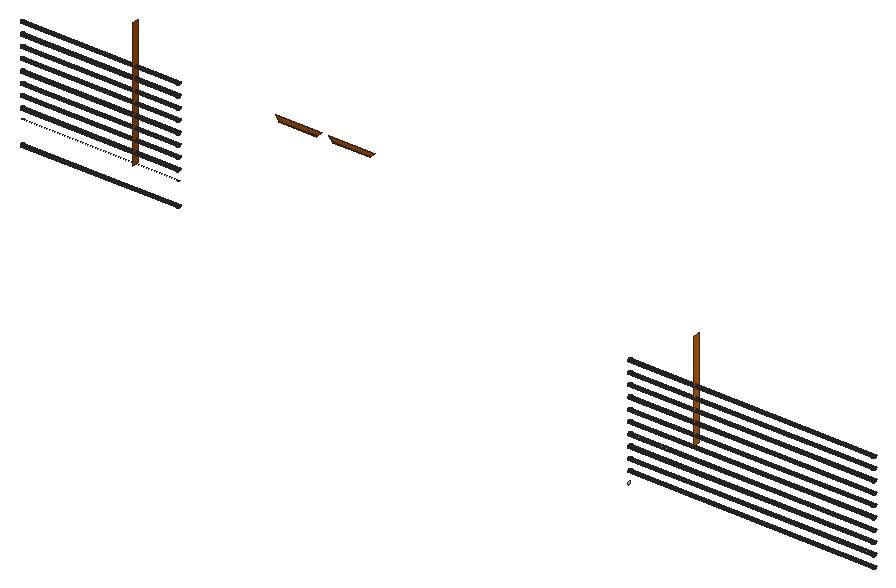
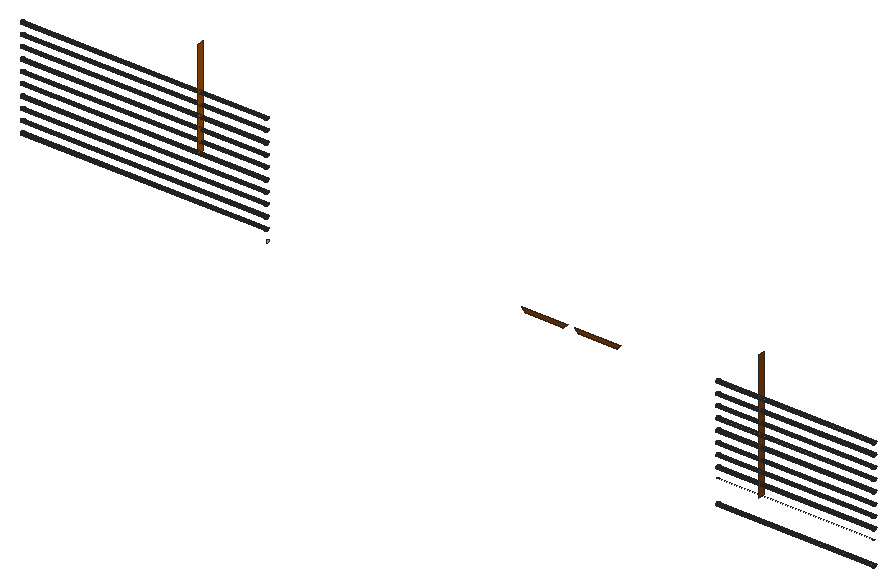
# SketchUp Ruby script. Lengths in inches.
U = 1.inch
M = Sketchup.active_model
def pt(a) = Geom::Point3d.new(a.map { |v| v * U })
def face(e, loops, mat)
  f = e.add_face(loops[0].map { |a| pt(a) })
  loops[1..].each { |l| e.add_face(l.map { |a| pt(a) }).erase! }
  f.material = f.back_material = mat if mat
  f
end
# faces: each face lists its corners as indices into pts; further lists are holes
def faces(e, pts, list, mat = nil) = list.each { |f| face(e, (f[0].is_a?(Array) ? f : [f]).map { |l| l.map { |i| pts[i] } }, mat) }
# xy, xz, yz: faces in a plane at the given z, y or x. An outline is a flat list of corners, or four numbers for a rectangle; further outlines are holes
def ring(l) = l.size == 4 ? [[l[0], l[1]], [l[2], l[1]], [l[2], l[3]], [l[0], l[3]]] : l.each_slice(2).to_a
def flat(e, list, mat, &to3) = list.each { |f| face(e, (f[0].is_a?(Array) ? f : [f]).map { |l| ring(l).map { |u, v| to3.(u, v) } }, mat) }
def xy(e, z, list, mat = nil) = flat(e, list, mat) { |x, y| [x, y, z] }
def xz(e, y, list, mat = nil) = flat(e, list, mat) { |x, z| [x, y, z] }
def yz(e, x, list, mat = nil) = flat(e, list, mat) { |y, z| [x, y, z] }
def lines(e, pts, list) = list.each { |a, b| e.add_line(pt(pts[a]), pt(pts[b])) }
# prism: a flat outline (further loops are holes) pulled along v
def prism(e, loops, v, mat = nil)
  f = face(e, loops, mat); d = Geom::Vector3d.new(v.map { |x| x * U })
  f.pushpull(f.normal.samedirection?(d) ? d.length : -d.length)
end
def box(e, o, s, mat = nil) = prism(e, [[o, [o[0] + s[0], o[1], o[2]], [o[0] + s[0], o[1] + s[1], o[2]], [o[0], o[1] + s[1], o[2]]]], [0, 0, s[2]], mat)
def at(x, y, z, deg = 0) = Geom::Transformation.translation(pt([x, y, z])) * Geom::Transformation.rotation(ORIGIN, Z_AXIS, deg.degrees)
def axes(o, x, y, z) = Geom::Transformation.new([*x, 0, *y, 0, *z, 0, *pt(o).to_a, 1])
def part(name) = M.definitions.add(name)
# library, detail: a bought-in or finely detailed component or shape, given as its bounding box
def library(name, o, s) = part(name).tap { |d| box(d.entities, o, s) }
def detail(e, o, s) = box(e.add_group.entities, o, s)
def put(e, d, t, mat = nil) = e.add_instance(d, t).tap { |i| i.material = mat if mat }
def group(e, t, mat = nil) = e.add_group.tap { |g| g.transformation = t; g.material = mat if mat }.entities
root = M.entities
M.materials.add("[0132_LightGray]").color = [169, 169, 169]
M.materials.add("[Wood Bamboo]").color = [195, 96, 5]
M.materials.add("[Wood Cherry Original]").color = [152, 68, 0]
xy(root,121.5,[[154,85.05,167.69,85.25],[173.29,85.05,186.99,85.25]])
xz(root,85.25,[[154,121.5,167.69,121.5,169.19,123,152.5,123],[173.29,121.5,186.99,121.5,188.49,123,171.79,123]],"[Wood Cherry Original]")
yz(root,103.25,[[82.25,90.51,84.25,137.01]],"[Wood Cherry Original]")
yz(root,316.01,[[41.28,79.71,41.15,79.73,41.03,79.78,40.93,79.86,40.85,79.96,40.8,80.08,40.78,80.21,40.8,80.34,40.85,80.46,40.93,80.57,41.03,80.65,41.15,80.7,41.28,80.71,41.41,80.7,41.53,80.65,41.63,80.57,41.71,80.46,41.76,80.34,41.78,80.21,41.76,80.08,41.71,79.96,41.63,79.86,41.53,79.78,41.41,79.73]])
yz(root,340.01,[[40.5625,100.9,43,136.59]],"[Wood Bamboo]")
p = [[119.25,83,82.03],[119.25,82.9,82.11],[61.9375,82.9,82.11],[61.9375,83,82.03],[119.25,83.12,81.98],[61.9375,83.12,81.98],
  [119.25,83.25,81.96],[61.9375,83.25,81.96],[119.25,83.38,81.98],[61.9375,83.38,81.98],[119.25,83.5,82.03],[61.9375,83.5,82.03],
  [119.25,83.6,82.11],[61.9375,83.6,82.11],[119.25,82.82,82.21],[61.9375,82.82,82.21],[119.25,83.68,82.21],[61.9375,83.68,82.21],
  [119.25,82.77,82.34],[61.9375,82.77,82.34],[119.25,83.73,82.34],[61.9375,83.73,82.34],[119.25,82.75,82.46],[61.9375,82.75,82.46],
  [119.25,83.75,82.46],[61.9375,83.75,82.46],[119.25,82.77,82.59],[61.9375,82.77,82.59],[119.25,83.73,82.59],[61.9375,83.73,82.59],
  [119.25,82.82,82.71],[61.9375,82.82,82.71],[119.25,83.68,82.71],[61.9375,83.68,82.71],[119.25,82.9,82.82],[61.9375,82.9,82.82],
  [119.25,83.6,82.82],[61.9375,83.6,82.82],[119.25,83,82.9],[61.9375,83,82.9],[119.25,83.5,82.9],[61.9375,83.5,82.9],
  [119.25,83.12,82.95],[61.9375,83.12,82.95],[119.25,83.25,82.96],[61.9375,83.25,82.96],[119.25,83.38,82.95],[61.9375,83.38,82.95],
  [316.01,41.03,83.78],[316.01,41.15,83.73],[405.26,41.15,83.73],[405.26,41.03,83.78],[316.01,41.28,83.71],[405.26,41.28,83.71],
  [316.01,41.41,83.73],[405.26,41.41,83.73],[316.01,41.53,83.78],[405.26,41.53,83.78],[316.01,40.93,83.86],[405.26,40.93,83.86],
  [316.01,41.63,83.86],[405.26,41.63,83.86],[316.01,40.85,83.96],[405.26,40.85,83.96],[316.01,41.71,83.96],[405.26,41.71,83.96],
  [316.01,40.8,84.08],[405.26,40.8,84.08],[316.01,41.76,84.08],[405.26,41.76,84.08],[316.01,40.78,84.21],[405.26,40.78,84.21],
  [316.01,41.78,84.21],[405.26,41.78,84.21],[316.01,40.8,84.34],[405.26,40.8,84.34],[316.01,41.76,84.34],[405.26,41.76,84.34],
  [316.01,40.85,84.46],[405.26,40.85,84.46],[316.01,41.71,84.46],[405.26,41.71,84.46],[316.01,40.93,84.57],[405.26,40.93,84.57],
  [316.01,41.63,84.57],[405.26,41.63,84.57],[316.01,41.03,84.65],[405.26,41.03,84.65],[316.01,41.15,84.7],[405.26,41.15,84.7],
  [316.01,41.53,84.65],[316.01,41.41,84.7],[405.26,41.41,84.7],[405.26,41.53,84.65],[316.01,41.28,84.71],[405.26,41.28,84.71],
  [316.01,41.03,87.78],[316.01,41.15,87.73],[405.26,41.15,87.73],[405.26,41.03,87.78],[316.01,41.28,87.71],[405.26,41.28,87.71],
  [316.01,41.41,87.73],[405.26,41.41,87.73],[316.01,41.53,87.78],[405.26,41.53,87.78],[316.01,40.93,87.86],[405.26,40.93,87.86],
  [316.01,41.63,87.86],[405.26,41.63,87.86],[316.01,40.85,87.96],[405.26,40.85,87.96],[316.01,41.71,87.96],[405.26,41.71,87.96],
  [316.01,40.8,88.08],[405.26,40.8,88.08],[316.01,41.76,88.08],[405.26,41.76,88.08],[316.01,40.78,88.21],[405.26,40.78,88.21],
  [316.01,41.78,88.21],[405.26,41.78,88.21],[316.01,40.8,88.34],[405.26,40.8,88.34],[316.01,41.76,88.34],[405.26,41.76,88.34],
  [316.01,40.85,88.46],[405.26,40.85,88.46],[316.01,41.71,88.46],[405.26,41.71,88.46],[316.01,40.93,88.57],[405.26,40.93,88.57],
  [316.01,41.63,88.57],[405.26,41.63,88.57],[316.01,41.03,88.65],[405.26,41.03,88.65],[316.01,41.15,88.7],[405.26,41.15,88.7],
  [316.01,41.53,88.65],[316.01,41.41,88.7],[405.26,41.41,88.7],[405.26,41.53,88.65],[316.01,41.28,88.71],[405.26,41.28,88.71],
  [119.25,83.25,90.96],[119.25,83.38,90.95],[61.9375,83.38,90.95],[61.9375,83.25,90.96],[316.01,41.03,91.78],[316.01,41.15,91.73],
  [405.26,41.15,91.73],[405.26,41.03,91.78],[316.01,41.28,91.71],[405.26,41.28,91.71],[316.01,41.41,91.73],[405.26,41.41,91.73],
  [316.01,41.53,91.78],[405.26,41.53,91.78],[316.01,40.93,91.86],[405.26,40.93,91.86],[316.01,41.63,91.86],[405.26,41.63,91.86],
  [316.01,40.85,91.96],[405.26,40.85,91.96],[316.01,41.71,91.96],[405.26,41.71,91.96],[316.01,40.8,92.08],[405.26,40.8,92.08],
  [316.01,41.76,92.08],[405.26,41.76,92.08],[316.01,40.78,92.21],[405.26,40.78,92.21],[316.01,41.78,92.21],[405.26,41.78,92.21],
  [316.01,40.8,92.34],[405.26,40.8,92.34],[316.01,41.76,92.34],[405.26,41.76,92.34],[316.01,40.85,92.46],[405.26,40.85,92.46],
  [316.01,41.71,92.46],[405.26,41.71,92.46],[316.01,40.93,92.57],[405.26,40.93,92.57],[316.01,41.63,92.57],[405.26,41.63,92.57],
  [316.01,41.03,92.65],[405.26,41.03,92.65],[316.01,41.15,92.7],[405.26,41.15,92.7],[316.01,41.53,92.65],[316.01,41.41,92.7],
  [405.26,41.41,92.7],[405.26,41.53,92.65],[316.01,41.28,92.71],[405.26,41.28,92.71],[119.25,83,94.03],[119.25,82.9,94.11],
  [61.9375,82.9,94.11],[61.9375,83,94.03],[119.25,83.12,93.98],[61.9375,83.12,93.98],[119.25,83.25,93.96],[61.9375,83.25,93.96],
  [119.25,83.38,93.98],[61.9375,83.38,93.98],[119.25,83.5,94.03],[61.9375,83.5,94.03],[119.25,83.6,94.11],[61.9375,83.6,94.11],
  [119.25,82.82,94.21],[61.9375,82.82,94.21],[119.25,83.68,94.21],[61.9375,83.68,94.21],[119.25,82.77,94.34],[61.9375,82.77,94.34],
  [119.25,83.73,94.34],[61.9375,83.73,94.34],[119.25,82.75,94.46],[61.9375,82.75,94.46],[119.25,83.75,94.46],[61.9375,83.75,94.46],
  [119.25,82.77,94.59],[61.9375,82.77,94.59],[119.25,83.73,94.59],[61.9375,83.73,94.59],[119.25,82.82,94.71],[61.9375,82.82,94.71],
  [119.25,83.68,94.71],[61.9375,83.68,94.71],[119.25,82.9,94.82],[61.9375,82.9,94.82],[119.25,83.6,94.82],[61.9375,83.6,94.82],
  [119.25,83,94.9],[61.9375,83,94.9],[119.25,83.5,94.9],[61.9375,83.5,94.9],[119.25,83.12,94.95],[61.9375,83.12,94.95],
  [119.25,83.25,94.96],[61.9375,83.25,94.96],[119.25,83.38,94.95],[61.9375,83.38,94.95],[316.01,41.03,95.78],[316.01,41.15,95.73],
  [405.26,41.15,95.73],[405.26,41.03,95.78],[316.01,41.28,95.71],[405.26,41.28,95.71],[316.01,41.41,95.73],[405.26,41.41,95.73],
  [316.01,41.53,95.78],[405.26,41.53,95.78],[316.01,40.93,95.86],[405.26,40.93,95.86],[316.01,41.63,95.86],[405.26,41.63,95.86],
  [316.01,40.85,95.96],[405.26,40.85,95.96],[316.01,41.71,95.96],[405.26,41.71,95.96],[316.01,40.8,96.08],[405.26,40.8,96.08],
  [316.01,41.76,96.08],[405.26,41.76,96.08],[316.01,40.78,96.21],[405.26,40.78,96.21],[316.01,41.78,96.21],[405.26,41.78,96.21],
  [316.01,40.8,96.34],[405.26,40.8,96.34],[316.01,41.76,96.34],[405.26,41.76,96.34],[316.01,40.85,96.46],[405.26,40.85,96.46],
  [316.01,41.71,96.46],[405.26,41.71,96.46],[316.01,40.93,96.57],[405.26,40.93,96.57],[316.01,41.63,96.57],[405.26,41.63,96.57],
  [316.01,41.03,96.65],[405.26,41.03,96.65],[316.01,41.15,96.7],[405.26,41.15,96.7],[316.01,41.53,96.65],[316.01,41.41,96.7],
  [405.26,41.41,96.7],[405.26,41.53,96.65],[316.01,41.28,96.71],[405.26,41.28,96.71],[119.25,83,98.03],[119.25,82.9,98.11],
  [61.9375,82.9,98.11],[61.9375,83,98.03],[119.25,83.12,97.98],[61.9375,83.12,97.98],[119.25,83.25,97.96],[61.9375,83.25,97.96],
  [119.25,83.38,97.98],[61.9375,83.38,97.98],[119.25,83.5,98.03],[61.9375,83.5,98.03],[119.25,83.6,98.11],[61.9375,83.6,98.11],
  [119.25,82.82,98.21],[61.9375,82.82,98.21],[119.25,83.68,98.21],[61.9375,83.68,98.21],[119.25,82.77,98.34],[61.9375,82.77,98.34],
  [119.25,83.73,98.34],[61.9375,83.73,98.34],[119.25,82.75,98.46],[61.9375,82.75,98.46],[119.25,83.75,98.46],[61.9375,83.75,98.46],
  [119.25,82.77,98.59],[61.9375,82.77,98.59],[119.25,83.73,98.59],[61.9375,83.73,98.59],[119.25,82.82,98.71],[61.9375,82.82,98.71],
  [119.25,83.68,98.71],[61.9375,83.68,98.71],[119.25,82.9,98.82],[61.9375,82.9,98.82],[119.25,83.6,98.82],[61.9375,83.6,98.82],
  [119.25,83,98.9],[61.9375,83,98.9],[119.25,83.5,98.9],[61.9375,83.5,98.9],[119.25,83.12,98.95],[61.9375,83.12,98.95],
  [119.25,83.25,98.96],[61.9375,83.25,98.96],[119.25,83.38,98.95],[61.9375,83.38,98.95],[316.01,41.03,99.78],[316.01,41.15,99.73],
  [405.26,41.15,99.73],[405.26,41.03,99.78],[316.01,41.28,99.71],[405.26,41.28,99.71],[316.01,41.41,99.73],[405.26,41.41,99.73],
  [316.01,41.53,99.78],[405.26,41.53,99.78],[316.01,40.93,99.86],[405.26,40.93,99.86],[316.01,41.63,99.86],[405.26,41.63,99.86],
  [316.01,40.85,99.96],[405.26,40.85,99.96],[316.01,41.71,99.96],[405.26,41.71,99.96],[316.01,40.8,100.08],[405.26,40.8,100.08],
  [316.01,41.76,100.08],[405.26,41.76,100.08],[316.01,40.78,100.21],[405.26,40.78,100.21],[316.01,41.78,100.21],[405.26,41.78,100.21],
  [316.01,40.8,100.34],[405.26,40.8,100.34],[316.01,41.76,100.34],[405.26,41.76,100.34],[316.01,40.85,100.46],[405.26,40.85,100.46],
  [316.01,41.71,100.46],[405.26,41.71,100.46],[316.01,40.93,100.57],[405.26,40.93,100.57],[316.01,41.63,100.57],[405.26,41.63,100.57],
  [316.01,41.03,100.65],[405.26,41.03,100.65],[316.01,41.15,100.7],[405.26,41.15,100.7],[316.01,41.53,100.65],[316.01,41.41,100.7],
  [405.26,41.41,100.7],[405.26,41.53,100.65],[316.01,41.28,100.71],[405.26,41.28,100.71],[119.25,83,102.03],[119.25,82.9,102.11],
  [61.9375,82.9,102.11],[61.9375,83,102.03],[119.25,83.12,101.98],[61.9375,83.12,101.98],[119.25,83.25,101.96],[61.9375,83.25,101.96],
  [119.25,83.38,101.98],[61.9375,83.38,101.98],[119.25,83.5,102.03],[61.9375,83.5,102.03],[119.25,83.6,102.11],[61.9375,83.6,102.11],
  [119.25,82.82,102.21],[61.9375,82.82,102.21],[119.25,83.68,102.21],[61.9375,83.68,102.21],[119.25,82.77,102.34],[61.9375,82.77,102.34],
  [119.25,83.73,102.34],[61.9375,83.73,102.34],[119.25,82.75,102.46],[61.9375,82.75,102.46],[119.25,83.75,102.46],[61.9375,83.75,102.46],
  [119.25,82.77,102.59],[61.9375,82.77,102.59],[119.25,83.73,102.59],[61.9375,83.73,102.59],[119.25,82.82,102.71],[61.9375,82.82,102.71],
  [119.25,83.68,102.71],[61.9375,83.68,102.71],[119.25,82.9,102.82],[61.9375,82.9,102.82],[119.25,83.6,102.82],[61.9375,83.6,102.82],
  [119.25,83,102.9],[61.9375,83,102.9],[119.25,83.5,102.9],[61.9375,83.5,102.9],[119.25,83.12,102.95],[61.9375,83.12,102.95],
  [119.25,83.25,102.96],[61.9375,83.25,102.96],[119.25,83.38,102.95],[61.9375,83.38,102.95],[316.01,41.03,103.78],[316.01,41.15,103.73],
  [405.26,41.15,103.73],[405.26,41.03,103.78],[316.01,41.28,103.71],[405.26,41.28,103.71],[316.01,41.41,103.73],[405.26,41.41,103.73],
  [316.01,41.53,103.78],[405.26,41.53,103.78],[316.01,40.93,103.86],[405.26,40.93,103.86],[316.01,41.63,103.86],[405.26,41.63,103.86],
  [316.01,40.85,103.96],[405.26,40.85,103.96],[316.01,41.71,103.96],[405.26,41.71,103.96],[316.01,40.8,104.08],[405.26,40.8,104.08],
  [316.01,41.76,104.08],[405.26,41.76,104.08],[316.01,40.78,104.21],[405.26,40.78,104.21],[316.01,41.78,104.21],[405.26,41.78,104.21],
  [316.01,40.8,104.34],[405.26,40.8,104.34],[316.01,41.76,104.34],[405.26,41.76,104.34],[316.01,40.85,104.46],[405.26,40.85,104.46],
  [316.01,41.71,104.46],[405.26,41.71,104.46],[316.01,40.93,104.57],[405.26,40.93,104.57],[316.01,41.63,104.57],[405.26,41.63,104.57],
  [316.01,41.03,104.65],[405.26,41.03,104.65],[316.01,41.15,104.7],[405.26,41.15,104.7],[316.01,41.53,104.65],[316.01,41.41,104.7],
  [405.26,41.41,104.7],[405.26,41.53,104.65],[316.01,41.28,104.71],[405.26,41.28,104.71],[119.25,83,106.03],[119.25,82.9,106.11],
  [61.9375,82.9,106.11],[61.9375,83,106.03],[119.25,83.12,105.98],[61.9375,83.12,105.98],[119.25,83.25,105.96],[61.9375,83.25,105.96],
  [119.25,83.38,105.98],[61.9375,83.38,105.98],[119.25,83.5,106.03],[61.9375,83.5,106.03],[119.25,83.6,106.11],[61.9375,83.6,106.11],
  [119.25,82.82,106.21],[61.9375,82.82,106.21],[119.25,83.68,106.21],[61.9375,83.68,106.21],[119.25,82.77,106.34],[61.9375,82.77,106.34],
  [119.25,83.73,106.34],[61.9375,83.73,106.34],[119.25,82.75,106.46],[61.9375,82.75,106.46],[119.25,83.75,106.46],[61.9375,83.75,106.46],
  [119.25,82.77,106.59],[61.9375,82.77,106.59],[119.25,83.73,106.59],[61.9375,83.73,106.59],[119.25,82.82,106.71],[61.9375,82.82,106.71],
  [119.25,83.68,106.71],[61.9375,83.68,106.71],[119.25,82.9,106.82],[61.9375,82.9,106.82],[119.25,83.6,106.82],[61.9375,83.6,106.82],
  [119.25,83,106.9],[61.9375,83,106.9],[119.25,83.5,106.9],[61.9375,83.5,106.9],[119.25,83.12,106.95],[61.9375,83.12,106.95],
  [119.25,83.25,106.96],[61.9375,83.25,106.96],[119.25,83.38,106.95],[61.9375,83.38,106.95],[316.01,41.03,107.78],[316.01,41.15,107.73],
  [405.26,41.15,107.73],[405.26,41.03,107.78],[316.01,41.28,107.71],[405.26,41.28,107.71],[316.01,41.41,107.73],[405.26,41.41,107.73],
  [316.01,41.53,107.78],[405.26,41.53,107.78],[316.01,40.93,107.86],[405.26,40.93,107.86],[316.01,41.63,107.86],[405.26,41.63,107.86],
  [316.01,40.85,107.96],[405.26,40.85,107.96],[316.01,41.71,107.96],[405.26,41.71,107.96],[316.01,40.8,108.08],[405.26,40.8,108.08],
  [316.01,41.76,108.08],[405.26,41.76,108.08],[316.01,40.78,108.21],[405.26,40.78,108.21],[316.01,41.78,108.21],[405.26,41.78,108.21],
  [316.01,40.8,108.34],[405.26,40.8,108.34],[316.01,41.76,108.34],[405.26,41.76,108.34],[316.01,40.85,108.46],[405.26,40.85,108.46],
  [316.01,41.71,108.46],[405.26,41.71,108.46],[316.01,40.93,108.57],[405.26,40.93,108.57],[316.01,41.63,108.57],[405.26,41.63,108.57],
  [316.01,41.03,108.65],[405.26,41.03,108.65],[316.01,41.15,108.7],[405.26,41.15,108.7],[316.01,41.53,108.65],[316.01,41.41,108.7],
  [405.26,41.41,108.7],[405.26,41.53,108.65],[316.01,41.28,108.71],[405.26,41.28,108.71],[119.25,83,110.03],[119.25,82.9,110.11],
  [61.9375,82.9,110.11],[61.9375,83,110.03],[119.25,83.12,109.98],[61.9375,83.12,109.98],[119.25,83.25,109.96],[61.9375,83.25,109.96],
  [119.25,83.38,109.98],[61.9375,83.38,109.98],[119.25,83.5,110.03],[61.9375,83.5,110.03],[119.25,83.6,110.11],[61.9375,83.6,110.11],
  [119.25,82.82,110.21],[61.9375,82.82,110.21],[119.25,83.68,110.21],[61.9375,83.68,110.21],[119.25,82.77,110.34],[61.9375,82.77,110.34],
  [119.25,83.73,110.34],[61.9375,83.73,110.34],[119.25,82.75,110.46],[61.9375,82.75,110.46],[119.25,83.75,110.46],[61.9375,83.75,110.46],
  [119.25,82.77,110.59],[61.9375,82.77,110.59],[119.25,83.73,110.59],[61.9375,83.73,110.59],[119.25,82.82,110.71],[61.9375,82.82,110.71],
  [119.25,83.68,110.71],[61.9375,83.68,110.71],[119.25,82.9,110.82],[61.9375,82.9,110.82],[119.25,83.6,110.82],[61.9375,83.6,110.82],
  [119.25,83,110.9],[61.9375,83,110.9],[119.25,83.5,110.9],[61.9375,83.5,110.9],[119.25,83.12,110.95],[61.9375,83.12,110.95],
  [119.25,83.25,110.96],[61.9375,83.25,110.96],[119.25,83.38,110.95],[61.9375,83.38,110.95],[316.01,41.03,111.78],[316.01,41.15,111.73],
  [405.26,41.15,111.73],[405.26,41.03,111.78],[316.01,41.28,111.71],[405.26,41.28,111.71],[316.01,41.41,111.73],[405.26,41.41,111.73],
  [316.01,41.53,111.78],[405.26,41.53,111.78],[316.01,40.93,111.86],[405.26,40.93,111.86],[316.01,41.63,111.86],[405.26,41.63,111.86],
  [316.01,40.85,111.96],[405.26,40.85,111.96],[316.01,41.71,111.96],[405.26,41.71,111.96],[316.01,40.8,112.08],[405.26,40.8,112.08],
  [316.01,41.76,112.08],[405.26,41.76,112.08],[316.01,40.78,112.21],[405.26,40.78,112.21],[316.01,41.78,112.21],[405.26,41.78,112.21],
  [316.01,40.8,112.34],[405.26,40.8,112.34],[316.01,41.76,112.34],[405.26,41.76,112.34],[316.01,40.85,112.46],[405.26,40.85,112.46],
  [316.01,41.71,112.46],[405.26,41.71,112.46],[316.01,40.93,112.57],[405.26,40.93,112.57],[316.01,41.63,112.57],[405.26,41.63,112.57],
  [316.01,41.03,112.65],[405.26,41.03,112.65],[316.01,41.15,112.7],[405.26,41.15,112.7],[316.01,41.53,112.65],[316.01,41.41,112.7],
  [405.26,41.41,112.7],[405.26,41.53,112.65],[316.01,41.28,112.71],[405.26,41.28,112.71],[119.25,83,114.03],[119.25,82.9,114.11],
  [61.9375,82.9,114.11],[61.9375,83,114.03],[119.25,83.12,113.98],[61.9375,83.12,113.98],[119.25,83.25,113.96],[61.9375,83.25,113.96],
  [119.25,83.38,113.98],[61.9375,83.38,113.98],[119.25,83.5,114.03],[61.9375,83.5,114.03],[119.25,83.6,114.11],[61.9375,83.6,114.11],
  [119.25,82.82,114.21],[61.9375,82.82,114.21],[119.25,83.68,114.21],[61.9375,83.68,114.21],[119.25,82.77,114.34],[61.9375,82.77,114.34],
  [119.25,83.73,114.34],[61.9375,83.73,114.34],[119.25,82.75,114.46],[61.9375,82.75,114.46],[119.25,83.75,114.46],[61.9375,83.75,114.46],
  [119.25,82.77,114.59],[61.9375,82.77,114.59],[119.25,83.73,114.59],[61.9375,83.73,114.59],[119.25,82.82,114.71],[61.9375,82.82,114.71],
  [119.25,83.68,114.71],[61.9375,83.68,114.71],[119.25,82.9,114.82],[61.9375,82.9,114.82],[119.25,83.6,114.82],[61.9375,83.6,114.82],
  [119.25,83,114.9],[61.9375,83,114.9],[119.25,83.5,114.9],[61.9375,83.5,114.9],[119.25,83.12,114.95],[61.9375,83.12,114.95],
  [119.25,83.25,114.96],[61.9375,83.25,114.96],[119.25,83.38,114.95],[61.9375,83.38,114.95],[316.01,41.03,115.78],[316.01,41.15,115.73],
  [405.26,41.15,115.73],[405.26,41.03,115.78],[316.01,41.28,115.71],[405.26,41.28,115.71],[316.01,41.41,115.73],[405.26,41.41,115.73],
  [316.01,41.53,115.78],[405.26,41.53,115.78],[316.01,40.93,115.86],[405.26,40.93,115.86],[316.01,41.63,115.86],[405.26,41.63,115.86],
  [316.01,40.85,115.96],[405.26,40.85,115.96],[316.01,41.71,115.96],[405.26,41.71,115.96],[316.01,40.8,116.08],[405.26,40.8,116.08],
  [316.01,41.76,116.08],[405.26,41.76,116.08],[316.01,40.78,116.21],[405.26,40.78,116.21],[316.01,41.78,116.21],[405.26,41.78,116.21],
  [316.01,40.8,116.34],[405.26,40.8,116.34],[316.01,41.76,116.34],[405.26,41.76,116.34],[316.01,40.85,116.46],[405.26,40.85,116.46],
  [316.01,41.71,116.46],[405.26,41.71,116.46],[316.01,40.93,116.57],[405.26,40.93,116.57],[316.01,41.63,116.57],[405.26,41.63,116.57],
  [316.01,41.03,116.65],[405.26,41.03,116.65],[316.01,41.15,116.7],[405.26,41.15,116.7],[316.01,41.53,116.65],[316.01,41.41,116.7],
  [405.26,41.41,116.7],[405.26,41.53,116.65],[316.01,41.28,116.71],[405.26,41.28,116.71],[119.25,83,118.03],[119.25,82.9,118.11],
  [61.9375,82.9,118.11],[61.9375,83,118.03],[119.25,83.12,117.98],[61.9375,83.12,117.98],[119.25,83.25,117.96],[61.9375,83.25,117.96],
  [119.25,83.38,117.98],[61.9375,83.38,117.98],[119.25,83.5,118.03],[61.9375,83.5,118.03],[119.25,83.6,118.11],[61.9375,83.6,118.11],
  [119.25,82.82,118.21],[61.9375,82.82,118.21],[119.25,83.68,118.21],[61.9375,83.68,118.21],[119.25,82.77,118.34],[61.9375,82.77,118.34],
  [119.25,83.73,118.34],[61.9375,83.73,118.34],[119.25,82.75,118.46],[61.9375,82.75,118.46],[119.25,83.75,118.46],[61.9375,83.75,118.46],
  [119.25,82.77,118.59],[61.9375,82.77,118.59],[119.25,83.73,118.59],[61.9375,83.73,118.59],[119.25,82.82,118.71],[61.9375,82.82,118.71],
  [119.25,83.68,118.71],[61.9375,83.68,118.71],[119.25,82.9,118.82],[61.9375,82.9,118.82],[119.25,83.6,118.82],[61.9375,83.6,118.82],
  [119.25,83,118.9],[61.9375,83,118.9],[119.25,83.5,118.9],[61.9375,83.5,118.9],[119.25,83.12,118.95],[61.9375,83.12,118.95],
  [119.25,83.25,118.96],[61.9375,83.25,118.96],[119.25,83.38,118.95],[61.9375,83.38,118.95],[316.01,41.03,119.78],[316.01,41.15,119.73],
  [405.26,41.15,119.73],[405.26,41.03,119.78],[316.01,41.28,119.71],[405.26,41.28,119.71],[316.01,41.41,119.73],[405.26,41.41,119.73],
  [316.01,41.53,119.78],[405.26,41.53,119.78],[316.01,40.93,119.86],[405.26,40.93,119.86],[316.01,41.63,119.86],[405.26,41.63,119.86],
  [316.01,40.85,119.96],[405.26,40.85,119.96],[316.01,41.71,119.96],[405.26,41.71,119.96],[316.01,40.8,120.08],[405.26,40.8,120.08],
  [316.01,41.76,120.08],[405.26,41.76,120.08],[316.01,40.78,120.21],[405.26,40.78,120.21],[316.01,41.78,120.21],[405.26,41.78,120.21],
  [316.01,40.8,120.34],[405.26,40.8,120.34],[316.01,41.76,120.34],[405.26,41.76,120.34],[316.01,40.85,120.46],[405.26,40.85,120.46],
  [316.01,41.71,120.46],[405.26,41.71,120.46],[316.01,40.93,120.57],[405.26,40.93,120.57],[316.01,41.63,120.57],[405.26,41.63,120.57],
  [316.01,41.03,120.65],[405.26,41.03,120.65],[316.01,41.15,120.7],[405.26,41.15,120.7],[316.01,41.53,120.65],[316.01,41.41,120.7],
  [405.26,41.41,120.7],[405.26,41.53,120.65],[316.01,41.28,120.71],[405.26,41.28,120.71],[119.25,83,122.03],[119.25,82.9,122.11],
  [61.9375,82.9,122.11],[61.9375,83,122.03],[119.25,83.12,121.98],[61.9375,83.12,121.98],[119.25,83.25,121.96],[61.9375,83.25,121.96],
  [119.25,83.38,121.98],[61.9375,83.38,121.98],[119.25,83.5,122.03],[61.9375,83.5,122.03],[119.25,83.6,122.11],[61.9375,83.6,122.11],
  [119.25,82.82,122.21],[61.9375,82.82,122.21],[119.25,83.68,122.21],[61.9375,83.68,122.21],[119.25,82.77,122.34],[61.9375,82.77,122.34],
  [119.25,83.73,122.34],[61.9375,83.73,122.34],[119.25,82.75,122.46],[61.9375,82.75,122.46],[119.25,83.75,122.46],[61.9375,83.75,122.46],
  [119.25,82.77,122.59],[61.9375,82.77,122.59],[119.25,83.73,122.59],[61.9375,83.73,122.59],[119.25,82.82,122.71],[61.9375,82.82,122.71],
  [119.25,83.68,122.71],[61.9375,83.68,122.71],[119.25,82.9,122.82],[61.9375,82.9,122.82],[119.25,83.6,122.82],[61.9375,83.6,122.82],
  [119.25,83,122.9],[61.9375,83,122.9],[119.25,83.5,122.9],[61.9375,83.5,122.9],[119.25,83.12,122.95],[61.9375,83.12,122.95],
  [119.25,83.25,122.96],[61.9375,83.25,122.96],[119.25,83.38,122.95],[61.9375,83.38,122.95]]
faces(root,p,[[0,1,2,3],[4,0,3,5],[6,4,5,7],[8,6,7,9],[10,8,9,11],[12,10,11,13],[1,14,15,2],[16,12,13,17],
  [14,18,19,15],[20,16,17,21],[18,22,23,19],[24,20,21,25],[22,26,27,23],[28,24,25,29],[26,30,31,27],[32,28,29,33],
  [30,34,35,31],[36,32,33,37],[34,38,39,35],[40,36,37,41],[38,42,43,39],[42,44,45,43],[44,46,47,45],[46,40,41,47],
  [48,49,50,51],[49,52,53,50],[52,54,55,53],[54,56,57,55],[58,48,51,59],[56,60,61,57],[62,58,59,63],[60,64,65,61],
  [66,62,63,67],[64,68,69,65],[70,66,67,71],[68,72,73,69],[74,70,71,75],[72,76,77,73],[78,74,75,79],[76,80,81,77],
  [82,78,79,83],[80,84,85,81],[86,82,83,87],[88,86,87,89],[90,91,92,93],[84,90,93,85],[94,88,89,95],[91,94,95,92],
  [96,97,98,99],[97,100,101,98],[100,102,103,101],[102,104,105,103],[106,96,99,107],[104,108,109,105],[110,106,107,111],[108,112,113,109],
  [114,110,111,115],[112,116,117,113],[118,114,115,119],[116,120,121,117],[122,118,119,123],[120,124,125,121],[126,122,123,127],[124,128,129,125],
  [130,126,127,131],[128,132,133,129],[134,130,131,135],[136,134,135,137],[138,139,140,141],[132,138,141,133],[142,136,137,143],[139,142,143,140],
  [144,145,146,147],[148,149,150,151],[149,152,153,150],[152,154,155,153],[154,156,157,155],[158,148,151,159],[156,160,161,157],[162,158,159,163],
  [160,164,165,161],[166,162,163,167],[164,168,169,165],[170,166,167,171],[168,172,173,169],[174,170,171,175],[172,176,177,173],[178,174,175,179],
  [176,180,181,177],[182,178,179,183],[180,184,185,181],[186,182,183,187],[188,186,187,189],[190,191,192,193],[184,190,193,185],[194,188,189,195],
  [191,194,195,192],[196,197,198,199],[200,196,199,201],[202,200,201,203],[204,202,203,205],[206,204,205,207],[208,206,207,209],[197,210,211,198],
  [212,208,209,213],[210,214,215,211],[216,212,213,217],[214,218,219,215],[220,216,217,221],[218,222,223,219],[224,220,221,225],[222,226,227,223],
  [228,224,225,229],[226,230,231,227],[232,228,229,233],[230,234,235,231],[236,232,233,237],[234,238,239,235],[238,240,241,239],[240,242,243,241],
  [242,236,237,243],[244,245,246,247],[245,248,249,246],[248,250,251,249],[250,252,253,251],[254,244,247,255],[252,256,257,253],[258,254,255,259],
  [256,260,261,257],[262,258,259,263],[260,264,265,261],[266,262,263,267],[264,268,269,265],[270,266,267,271],[268,272,273,269],[274,270,271,275],
  [272,276,277,273],[278,274,275,279],[276,280,281,277],[282,278,279,283],[284,282,283,285],[286,287,288,289],[280,286,289,281],[290,284,285,291],
  [287,290,291,288],[292,293,294,295],[296,292,295,297],[298,296,297,299],[300,298,299,301],[302,300,301,303],[304,302,303,305],[293,306,307,294],
  [308,304,305,309],[306,310,311,307],[312,308,309,313],[310,314,315,311],[316,312,313,317],[314,318,319,315],[320,316,317,321],[318,322,323,319],
  [324,320,321,325],[322,326,327,323],[328,324,325,329],[326,330,331,327],[332,328,329,333],[330,334,335,331],[334,336,337,335],[336,338,339,337],
  [338,332,333,339],[340,341,342,343],[341,344,345,342],[344,346,347,345],[346,348,349,347],[350,340,343,351],[348,352,353,349],[354,350,351,355],
  [352,356,357,353],[358,354,355,359],[356,360,361,357],[362,358,359,363],[360,364,365,361],[366,362,363,367],[364,368,369,365],[370,366,367,371],
  [368,372,373,369],[374,370,371,375],[372,376,377,373],[378,374,375,379],[380,378,379,381],[382,383,384,385],[376,382,385,377],[386,380,381,387],
  [383,386,387,384],[388,389,390,391],[392,388,391,393],[394,392,393,395],[396,394,395,397],[398,396,397,399],[400,398,399,401],[389,402,403,390],
  [404,400,401,405],[402,406,407,403],[408,404,405,409],[406,410,411,407],[412,408,409,413],[410,414,415,411],[416,412,413,417],[414,418,419,415],
  [420,416,417,421],[418,422,423,419],[424,420,421,425],[422,426,427,423],[428,424,425,429],[426,430,431,427],[430,432,433,431],[432,434,435,433],
  [434,428,429,435],[436,437,438,439],[437,440,441,438],[440,442,443,441],[442,444,445,443],[446,436,439,447],[444,448,449,445],[450,446,447,451],
  [448,452,453,449],[454,450,451,455],[452,456,457,453],[458,454,455,459],[456,460,461,457],[462,458,459,463],[460,464,465,461],[466,462,463,467],
  [464,468,469,465],[470,466,467,471],[468,472,473,469],[474,470,471,475],[476,474,475,477],[478,479,480,481],[472,478,481,473],[482,476,477,483],
  [479,482,483,480],[484,485,486,487],[488,484,487,489],[490,488,489,491],[492,490,491,493],[494,492,493,495],[496,494,495,497],[485,498,499,486],
  [500,496,497,501],[498,502,503,499],[504,500,501,505],[502,506,507,503],[508,504,505,509],[506,510,511,507],[512,508,509,513],[510,514,515,511],
  [516,512,513,517],[514,518,519,515],[520,516,517,521],[518,522,523,519],[524,520,521,525],[522,526,527,523],[526,528,529,527],[528,530,531,529],
  [530,524,525,531],[532,533,534,535],[533,536,537,534],[536,538,539,537],[538,540,541,539],[542,532,535,543],[540,544,545,541],[546,542,543,547],
  [544,548,549,545],[550,546,547,551],[548,552,553,549],[554,550,551,555],[552,556,557,553],[558,554,555,559],[556,560,561,557],[562,558,559,563],
  [560,564,565,561],[566,562,563,567],[564,568,569,565],[570,566,567,571],[572,570,571,573],[574,575,576,577],[568,574,577,569],[578,572,573,579],
  [575,578,579,576],[580,581,582,583],[584,580,583,585],[586,584,585,587],[588,586,587,589],[590,588,589,591],[592,590,591,593],[581,594,595,582],
  [596,592,593,597],[594,598,599,595],[600,596,597,601],[598,602,603,599],[604,600,601,605],[602,606,607,603],[608,604,605,609],[606,610,611,607],
  [612,608,609,613],[610,614,615,611],[616,612,613,617],[614,618,619,615],[620,616,617,621],[618,622,623,619],[622,624,625,623],[624,626,627,625],
  [626,620,621,627],[628,629,630,631],[629,632,633,630],[632,634,635,633],[634,636,637,635],[638,628,631,639],[636,640,641,637],[642,638,639,643],
  [640,644,645,641],[646,642,643,647],[644,648,649,645],[650,646,647,651],[648,652,653,649],[654,650,651,655],[652,656,657,653],[658,654,655,659],
  [656,660,661,657],[662,658,659,663],[660,664,665,661],[666,662,663,667],[668,666,667,669],[670,671,672,673],[664,670,673,665],[674,668,669,675],
  [671,674,675,672],[676,677,678,679],[680,676,679,681],[682,680,681,683],[684,682,683,685],[686,684,685,687],[688,686,687,689],[677,690,691,678],
  [692,688,689,693],[690,694,695,691],[696,692,693,697],[694,698,699,695],[700,696,697,701],[698,702,703,699],[704,700,701,705],[702,706,707,703],
  [708,704,705,709],[706,710,711,707],[712,708,709,713],[710,714,715,711],[716,712,713,717],[714,718,719,715],[718,720,721,719],[720,722,723,721],
  [722,716,717,723],[724,725,726,727],[725,728,729,726],[728,730,731,729],[730,732,733,731],[734,724,727,735],[732,736,737,733],[738,734,735,739],
  [736,740,741,737],[742,738,739,743],[740,744,745,741],[746,742,743,747],[744,748,749,745],[750,746,747,751],[748,752,753,749],[754,750,751,755],
  [752,756,757,753],[758,754,755,759],[756,760,761,757],[762,758,759,763],[764,762,763,765],[766,767,768,769],[760,766,769,761],[770,764,765,771],
  [767,770,771,768],[772,773,774,775],[776,772,775,777],[778,776,777,779],[780,778,779,781],[782,780,781,783],[784,782,783,785],[773,786,787,774],
  [788,784,785,789],[786,790,791,787],[792,788,789,793],[790,794,795,791],[796,792,793,797],[794,798,799,795],[800,796,797,801],[798,802,803,799],
  [804,800,801,805],[802,806,807,803],[808,804,805,809],[806,810,811,807],[812,808,809,813],[810,814,815,811],[814,816,817,815],[816,818,819,817],
  [818,812,813,819],[820,821,822,823],[821,824,825,822],[824,826,827,825],[826,828,829,827],[830,820,823,831],[828,832,833,829],[834,830,831,835],
  [832,836,837,833],[838,834,835,839],[836,840,841,837],[842,838,839,843],[840,844,845,841],[846,842,843,847],[844,848,849,845],[850,846,847,851],
  [848,852,853,849],[854,850,851,855],[852,856,857,853],[858,854,855,859],[860,858,859,861],[862,863,864,865],[856,862,865,857],[866,860,861,867],
  [863,866,867,864],[868,869,870,871],[872,868,871,873],[874,872,873,875],[876,874,875,877],[878,876,877,879],[880,878,879,881],[869,882,883,870],
  [884,880,881,885],[882,886,887,883],[888,884,885,889],[886,890,891,887],[892,888,889,893],[890,894,895,891],[896,892,893,897],[894,898,899,895],
  [900,896,897,901],[898,902,903,899],[904,900,901,905],[902,906,907,903],[908,904,905,909],[906,910,911,907],[910,912,913,911],[912,914,915,913],
  [914,908,909,915]],"[0132_LightGray]")
